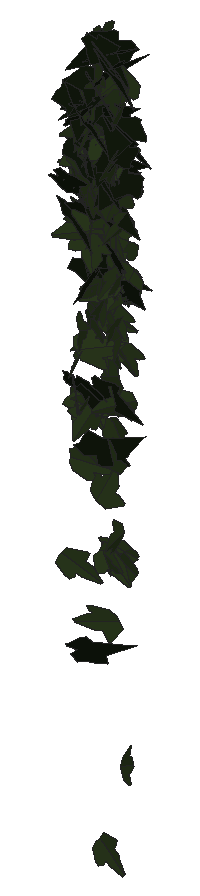
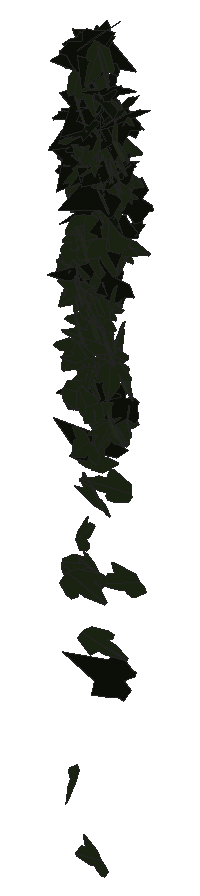
# SketchUp Ruby script. Lengths in inches.
U = 1.inch
M = Sketchup.active_model
def pt(a) = Geom::Point3d.new(a.map { |v| v * U })
def face(e, loops, mat)
  f = e.add_face(loops[0].map { |a| pt(a) })
  loops[1..].each { |l| e.add_face(l.map { |a| pt(a) }).erase! }
  f.material = f.back_material = mat if mat
  f
end
# faces: each face lists its corners as indices into pts; further lists are holes
def faces(e, pts, list, mat = nil) = list.each { |f| face(e, (f[0].is_a?(Array) ? f : [f]).map { |l| l.map { |i| pts[i] } }, mat) }
# xy, xz, yz: faces in a plane at the given z, y or x. An outline is a flat list of corners, or four numbers for a rectangle; further outlines are holes
def ring(l) = l.size == 4 ? [[l[0], l[1]], [l[2], l[1]], [l[2], l[3]], [l[0], l[3]]] : l.each_slice(2).to_a
def flat(e, list, mat, &to3) = list.each { |f| face(e, (f[0].is_a?(Array) ? f : [f]).map { |l| ring(l).map { |u, v| to3.(u, v) } }, mat) }
def xy(e, z, list, mat = nil) = flat(e, list, mat) { |x, y| [x, y, z] }
def xz(e, y, list, mat = nil) = flat(e, list, mat) { |x, z| [x, y, z] }
def yz(e, x, list, mat = nil) = flat(e, list, mat) { |y, z| [x, y, z] }
def lines(e, pts, list) = list.each { |a, b| e.add_line(pt(pts[a]), pt(pts[b])) }
# prism: a flat outline (further loops are holes) pulled along v
def prism(e, loops, v, mat = nil)
  f = face(e, loops, mat); d = Geom::Vector3d.new(v.map { |x| x * U })
  f.pushpull(f.normal.samedirection?(d) ? d.length : -d.length)
end
def box(e, o, s, mat = nil) = prism(e, [[o, [o[0] + s[0], o[1], o[2]], [o[0] + s[0], o[1] + s[1], o[2]], [o[0], o[1] + s[1], o[2]]]], [0, 0, s[2]], mat)
def at(x, y, z, deg = 0) = Geom::Transformation.translation(pt([x, y, z])) * Geom::Transformation.rotation(ORIGIN, Z_AXIS, deg.degrees)
def axes(o, x, y, z) = Geom::Transformation.new([*x, 0, *y, 0, *z, 0, *pt(o).to_a, 1])
def part(name) = M.definitions.add(name)
# library, detail: a bought-in or finely detailed component or shape, given as its bounding box
def library(name, o, s) = part(name).tap { |d| box(d.entities, o, s) }
def detail(e, o, s) = box(e.add_group.entities, o, s)
def put(e, d, t, mat = nil) = e.add_instance(d, t).tap { |i| i.material = mat if mat }
def group(e, t, mat = nil) = e.add_group.tap { |g| g.transformation = t; g.material = mat if mat }.entities
root = M.entities
M.materials.add("1026 AP 7946 SUNNY SIDE UP").color = [254, 231, 186]
M.materials.add("efeu1").color = [18, 25, 13]
M.materials.add("efeu2").color = [43, 57, 29]
c1 = part("ivyleaf_9")
p = [[1.54,2.16,1.25],[1.36,2.04,1.19],[-0.21,0.99,0.68],[-0.71,1.11,0.82],[-0.85,0.86,0.67],[-0.8,0.17,0.21],
  [-0.9,-0.01,0.1],[-0.67,-0.16,-0.02],[-0.08,-0.08,-0.05],[-0.03,-0.6,-0.4],[0.65,-0.88,-0.66],[0.83,-0.6,-0.49],
  [1.29,-0.42,-0.43],[1.8125,-0.07,-0.26],[1.21,0.44,0.15]]
faces(c1.entities,p,[[0,1,2,3,4,5,6,7,8,9,10,11,12,13,14]],"efeu1")
c2 = part("ivyleaf_10")
p = [[0,0.5,-0.03],[-0.0625,2.02,-0.43],[-0.19,2.01,-0.46],[-0.54,1.05,-0.29],[-0.52,0.625,-0.18],[-0.83,0.76,-0.28],
  [-1.16,0.64,-0.33],[-1.15,0.33,-0.24],[-0.77,-0.39,0.02],[-0.3,-0.51,0.16],[0.04,-0.48,0.23],[-0.02,2.01,-0.4375],
  [-0.06,2.01,-0.43],[0.04,-0.49,0.23],[0.67,-0.49,0.14],[1.38,0.36,-0.2],[1.375,0.51,-0.24],[0.81,0.65,-0.19],
  [0.62,0.59,-0.15],[0.6,1.09,-0.28],[0.5,1.23,-0.31]]
faces(c2.entities,p,[[0,1,2,3,4,5,6,7,8,9,10],[11,12,0,13,14,15,16,17,18,19,20]],"efeu2")
put(root,c1,axes([109.72,212.76,263.63],[0.13079,-0.20929,0.09165],[0.04808,-0.08485,-0.23249],[0.35508,0.08858,-0.00228]),"1026 AP 7946 SUNNY SIDE UP")
put(root,c2,axes([109.74,212.79,260.34],[0.07065,-0.07555,0.22326],[0.25364,-0.1473,-0.08805],[0.2576,0.16575,0.02546]),"1026 AP 7946 SUNNY SIDE UP")
put(root,c2,axes([109.94,212.7,261.06],[0.13125,-0.20202,0.03417],[0.00222,-0.03649,-0.22504],[0.32221,0.08255,-0.01237]),"1026 AP 7946 SUNNY SIDE UP")
put(root,c2,axes([109.89,212.84,264.64],[0.26049,0.1733,-0.05289],[-0.04276,-0.0463,-0.24695],[-0.28142,0.16745,-0.01144]),"1026 AP 7946 SUNNY SIDE UP")
put(root,c1,axes([109.86,212.83,265.76],[-0.08825,-0.23856,0.02828],[-0.00223,-0.02925,-0.25259],[0.37783,-0.0559,0.00512]),"1026 AP 7946 SUNNY SIDE UP")
put(root,c2,axes([110,212.6875,265.18],[0.18954,-0.20786,-0.07168],[-0.07557,0.05103,-0.24673],[0.33568,0.12886,-0.01508]),"1026 AP 7946 SUNNY SIDE UP")
put(root,c2,axes([110.16,212.74,263.43],[-0.1369,-0.00315,0.23171],[-0.24327,-0.17426,-0.06522],[0.25678,-0.16676,0.06174]),"1026 AP 7946 SUNNY SIDE UP")
put(root,c2,axes([109.96,212.96,261.23],[-0.12139,-0.20108,-0.05585],[0.03397,0.04854,-0.2216],[0.32524,-0.08012,0.0023]),"1026 AP 7946 SUNNY SIDE UP")
put(root,c1,axes([109.67,212.59,264.29],[0.36648,-0.04555,0.08565],[0.12006,-0.04172,-0.24355],[0.08895,0.244,-0.02413]),"1026 AP 7946 SUNNY SIDE UP")
put(root,c2,axes([109.97,212.83,265.22],[-0.195,-0.21529,-0.00433],[0.04409,-0.01274,-0.25407],[0.33567,-0.12339,0.03086]),"1026 AP 7946 SUNNY SIDE UP")
put(root,c2,axes([110.05,212.79,264.6],[-0.29975,-0.13813,0.05648],[-0.05119,-0.04948,-0.2419],[0.22846,-0.19231,0.0199]),"1026 AP 7946 SUNNY SIDE UP")
put(root,c2,axes([110.04,212.93,263.4375],[-0.31434,-0.10846,0.05691],[-0.0484,-0.05893,-0.23169],[0.18563,-0.19903,0.03597]),"1026 AP 7946 SUNNY SIDE UP")
put(root,c2,axes([109.83,212.97,265.43],[0.12638,-0.09056,0.21745],[0.18821,-0.17498,-0.12502],[0.30911,0.14357,-0.01278]),"1026 AP 7946 SUNNY SIDE UP")
put(root,c2,axes([109.97,212.9,264.94],[0.19883,-0.20933,-0.02797],[0.00715,0.03297,-0.25083],[0.33159,0.12481,0.02218]),"1026 AP 7946 SUNNY SIDE UP")
put(root,c2,axes([110.01,212.83,262.58],[-0.14678,0.20903,0.05276],[-0.07727,0.03234,-0.23348],[-0.329,-0.10085,0.0313]),"1026 AP 7946 SUNNY SIDE UP")
put(root,c1,axes([109.87,212.89,264.8],[0.01269,-0.2439,0.02232],[0.00005,-0.02306,-0.25153],[0.38522,0.00804,-0.0007]),"1026 AP 7946 SUNNY SIDE UP")
put(root,c2,axes([110.02,213,261.83],[0.1239,-0.20898,0.00095],[0.00598,-0.00082,-0.23007],[0.32857,0.07882,0.00383]),"1026 AP 7946 SUNNY SIDE UP")
put(root,c1,axes([109.81,212.83,265.95],[0.18215,-0.21944,-0.03716],[0.0086,0.04208,-0.25417],[0.34927,0.11341,0.02564]),"1026 AP 7946 SUNNY SIDE UP")
put(root,c2,axes([109.99,212.92,263.53],[-0.33875,0.07546,0.06254],[0.09273,-0.01392,0.23499],[0.12026,0.22328,-0.00503]),"1026 AP 7946 SUNNY SIDE UP")
put(root,c2,axes([110.02,212.76,260.19],[0.2646,0.12276,-0.07104],[-0.06702,-0.05913,-0.21379],[-0.21157,0.17226,-0.02112]),"1026 AP 7946 SUNNY SIDE UP")
put(root,c2,axes([110.19,212.78,265.2],[0.19235,-0.11093,-0.18515],[-0.20284,0.12428,-0.16935],[0.26188,0.17774,0.00482]),"1026 AP 7946 SUNNY SIDE UP")
put(root,c2,axes([110.09,212.73,263.49],[0.1737,-0.17874,-0.12958],[-0.05015,0.12512,-0.21301],[0.33906,0.11007,0.03488]),"1026 AP 7946 SUNNY SIDE UP")
put(root,c2,axes([110.06,212.86,264.89],[0.13038,-0.22595,0.05083],[0.01222,-0.05102,-0.24804],[0.36389,0.08267,-0.00988]),"1026 AP 7946 SUNNY SIDE UP")
put(root,c2,axes([110.07,212.77,260.25],[0.10919,-0.21636,0.03396],[0.00256,-0.03536,-0.23411],[0.34443,0.06886,-0.00903]),"1026 AP 7946 SUNNY SIDE UP")
put(root,c2,axes([110.01,212.75,264.88],[-0.12133,0.21466,-0.0854],[0.01343,-0.08598,-0.23462],[-0.36228,-0.07508,0.0199]),"1026 AP 7946 SUNNY SIDE UP")
put(root,c2,axes([110.06,212.56,264.42],[-0.31214,0.13505,-0.00457],[-0.01055,-0.01909,-0.24664],[-0.21225,-0.19766,0.01899]),"1026 AP 7946 SUNNY SIDE UP")
put(root,c1,axes([110.14,212.72,263.78],[0.24918,0.10255,-0.15469],[-0.21904,-0.06073,-0.19379],[-0.18493,0.21011,0.02111]),"1026 AP 7946 SUNNY SIDE UP")
put(root,c2,axes([110.14,212.8,261.67],[-0.24967,0.14445,0.06378],[-0.10517,0.01627,-0.21862],[-0.22307,-0.16935,0.03169]),"1026 AP 7946 SUNNY SIDE UP")
put(root,c2,axes([110.11,212.85,264.32],[-0.24381,-0.17738,0.06823],[0.0098,-0.09156,-0.23457],[0.29813,-0.14206,0.06351]),"1026 AP 7946 SUNNY SIDE UP")
put(root,c1,axes([109.9,212.82,265.01],[0.3859,0.01875,-0.00177],[-0.00389,0.00838,-0.25336],[-0.02937,0.24528,0.01023]),"1026 AP 7946 SUNNY SIDE UP")
put(root,c1,axes([109.83,212.9,264.9],[0.25725,-0.17887,0.03762],[0.04248,-0.02615,-0.24987],[0.28423,0.1658,0.0033]),"1026 AP 7946 SUNNY SIDE UP")
put(root,c1,axes([109.96,212.63,260.59],[0.37147,-0.01153,-0.0725],[-0.11178,-0.02184,-0.24251],[0.00751,0.24552,-0.02353]),"1026 AP 7946 SUNNY SIDE UP")
put(root,c1,axes([110.13,212.72,265.74],[0.19791,0.18578,-0.10609],[-0.08308,-0.08982,-0.23162],[-0.32432,0.13637,-0.0054]),"1026 AP 7946 SUNNY SIDE UP")
put(root,c2,axes([110.125,212.48,261.67],[0.07428,-0.10061,-0.21613],[0.01805,0.21426,-0.10222],[0.3646,0.00989,0.04909]),"1026 AP 7946 SUNNY SIDE UP")
put(root,c2,axes([109.85,212.55,257.27],[0.15202,0.03576,0.20935],[0.29884,0.07139,-0.10577],[-0.12554,0.21323,0.00172]),"1026 AP 7946 SUNNY SIDE UP")
put(root,c1,axes([110.11,212.52,265.66],[0.13967,0.21436,0.09141],[0.06154,0.07848,-0.23851],[-0.35882,0.0969,-0.00533]),"1026 AP 7946 SUNNY SIDE UP")
put(root,c2,axes([110.11,212.65,265.84],[0.31429,-0.15394,0.00427],[-0.0072,-0.01416,-0.25958],[0.24207,0.19944,-0.01327]),"1026 AP 7946 SUNNY SIDE UP")
put(root,c2,axes([110.15,212.72,260.01],[-0.11766,-0.16357,0.1602],[0.02148,-0.16772,-0.17492],[0.35523,-0.04403,0.06364]),"1026 AP 7946 SUNNY SIDE UP")
put(root,c2,axes([110.15,212.96,266.89],[0.18599,-0.21723,-0.05047],[-0.01253,0.04991,-0.25395],[0.34951,0.11739,0.01775]),"1026 AP 7946 SUNNY SIDE UP")
put(root,c2,axes([110.21,212.875,262.02],[0.22369,-0.12293,-0.14079],[-0.11804,0.11794,-0.19008],[0.26293,0.15753,0.03445]),"1026 AP 7946 SUNNY SIDE UP")
put(root,c2,axes([110.08,212.88,260.14],[0.05062,0.21389,0.0488],[0.00632,0.04606,-0.22255],[-0.34401,0.03232,0.00309]),"1026 AP 7946 SUNNY SIDE UP")
put(root,c1,axes([110.3,212.75,266.02],[-0.3004,0.11873,-0.1105],[0.07761,-0.1162,-0.22237],[-0.24008,-0.18613,0.06638]),"1026 AP 7946 SUNNY SIDE UP")
put(root,c2,axes([110.17,212.99,266.93],[-0.05677,-0.19428,-0.19837],[0.05551,0.18817,-0.20247],[0.42528,-0.0505,-0.00005]),"1026 AP 7946 SUNNY SIDE UP")
put(root,c2,axes([109.89,212.78,259.02],[-0.01548,0.0145,0.2404],[0.32924,0.10428,0.00304],[-0.16327,0.2089,-0.01667]),"1026 AP 7946 SUNNY SIDE UP")
put(root,c2,axes([110.1,212.86,264.7],[-0.28958,-0.14926,-0.07113],[0.16554,-0.02883,-0.22805],[0.19794,-0.19426,0.08667]),"1026 AP 7946 SUNNY SIDE UP")
put(root,c2,axes([110.22,212.89,264.62],[0.13468,-0.2271,-0.03328],[0.00031,0.03319,-0.24955],[0.36041,0.08483,0.01265]),"1026 AP 7946 SUNNY SIDE UP")
put(root,c2,axes([110.22,212.86,262.33],[-0.08569,-0.21964,-0.02362],[0.02689,0.01806,-0.23269],[0.346,-0.0558,0.01224]),"1026 AP 7946 SUNNY SIDE UP")
put(root,c2,axes([110.28,212.76,260.3125],[-0.25209,-0.14702,0.0398],[-0.03134,-0.03655,-0.22389],[0.23731,-0.16101,0.01271]),"1026 AP 7946 SUNNY SIDE UP")
put(root,c2,axes([110.43,212.85,256.2],[0.16178,-0.00491,-0.20985],[-0.31906,0.01802,-0.10594],[0.02876,0.22747,0.0052]),"1026 AP 7946 SUNNY SIDE UP")
put(root,c2,axes([110.25,212.89,265.07],[-0.18119,-0.21778,-0.01531],[0.02397,0.00733,-0.25358],[0.34227,-0.1158,0.00966]),"1026 AP 7946 SUNNY SIDE UP")
put(root,c1,axes([109.95,212.71,255.55],[0.2357,0.14291,-0.13636],[0.1064,0.11949,0.21125],[0.28814,-0.16102,0.03354]),"1026 AP 7946 SUNNY SIDE UP")
put(root,c2,axes([110.37,212.7,264.63],[-0.32201,0.07011,0.11018],[-0.18098,-0.0147,-0.218],[-0.08645,-0.23038,0.04597]),"1026 AP 7946 SUNNY SIDE UP")
put(root,c2,axes([110.26,212.74,266.51],[-0.24837,0.20213,-0.00499],[-0.0688,-0.04158,-0.25717],[-0.31043,-0.1525,0.06098]),"1026 AP 7946 SUNNY SIDE UP")
put(root,c2,axes([110.27,212.92,262.33],[-0.34788,0.04702,0.01628],[-0.02994,-0.01514,-0.2323],[-0.07188,-0.22127,0.01799]),"1026 AP 7946 SUNNY SIDE UP")
put(root,c2,axes([110.25,212.95,262.01],[0.05532,-0.22112,0.02292],[0.00046,-0.02375,-0.23077],[0.34964,0.03501,-0.00332]),"1026 AP 7946 SUNNY SIDE UP")
put(root,c2,axes([110.35,212.97,262.34],[0.12589,0.07172,-0.20639],[-0.22293,-0.14223,-0.11143],[-0.25032,0.16273,-0.00456]),"1026 AP 7946 SUNNY SIDE UP")
put(root,c1,axes([110.1,212.87,264.4],[0.21866,0.14211,0.1836],[0.19985,0.12382,-0.20409],[-0.29634,0.18837,-0.00216]),"1026 AP 7946 SUNNY SIDE UP")
put(root,c1,axes([110.22,212.91,266.17],[-0.18685,-0.22147,-0.01502],[0.03216,0.00411,-0.25837],[0.34738,-0.1195,0.01584]),"1026 AP 7946 SUNNY SIDE UP")
put(root,c1,axes([110.26,212.36,262.48],[0.0585,0.09433,0.24507],[0.12983,0.22253,-0.10315],[-0.38004,0.09054,0.00249]),"1026 AP 7946 SUNNY SIDE UP")
put(root,c1,axes([110.45,212.72,264.23],[-0.14774,0.22218,0.01512],[-0.03422,0.00532,-0.24779],[-0.34831,-0.09476,0.01793]),"1026 AP 7946 SUNNY SIDE UP")
put(root,c2,axes([110.32,212.82,263.27],[-0.27533,-0.15792,0.01302],[0.00199,-0.02156,-0.24242],[0.24921,-0.1743,0.01632]),"1026 AP 7946 SUNNY SIDE UP")
put(root,c1,axes([110.04,212.73,265.47],[0.19459,-0.20051,0.0869],[0.05342,-0.07937,-0.24289],[0.33855,0.12777,-0.01163]),"1026 AP 7946 SUNNY SIDE UP")
put(root,c2,axes([110.48,213.1875,257.37],[-0.18536,-0.09033,0.17569],[-0.19294,-0.11994,-0.15307],[0.23515,-0.16962,0.0129]),"1026 AP 7946 SUNNY SIDE UP")
put(root,c2,axes([110.35,212.88,262.45],[-0.20763,-0.19168,-0.0044],[0.01316,-0.0019,-0.23966],[0.30116,-0.13207,0.00744]),"1026 AP 7946 SUNNY SIDE UP")
put(root,c2,axes([110.1875,212.65,263.28],[0.36234,-0.00703,0.07593],[0.11395,-0.02864,-0.23626],[0.02418,0.24025,-0.02452]),"1026 AP 7946 SUNNY SIDE UP")
put(root,c2,axes([110.3,212.9,264.3],[0.26744,-0.17249,0.00507],[0.02904,0.00996,-0.24863],[0.26982,0.16989,0.02174]),"1026 AP 7946 SUNNY SIDE UP")
put(root,c2,axes([110.31,212.94,265.31],[-0.28185,0.15949,-0.04664],[0.02695,-0.04982,-0.24608],[-0.25969,-0.17827,0.02508]),"1026 AP 7946 SUNNY SIDE UP")
put(root,c2,axes([110.31,212.8,265.45],[0.21852,-0.1933,0.08066],[0.05455,-0.07268,-0.24529],[0.32402,0.1426,-0.0131]),"1026 AP 7946 SUNNY SIDE UP")
put(root,c1,axes([110.5,212.9375,266.96],[-0.03692,0.05146,-0.27915],[-0.02061,-0.27214,-0.05361],[-0.43365,0.00855,0.02632]),"1026 AP 7946 SUNNY SIDE UP")
put(root,c2,axes([110.42,212.91,266.25],[-0.14854,-0.22999,0.01109],[0.00153,-0.01344,-0.25615],[0.36213,-0.09428,0.00563]),"1026 AP 7946 SUNNY SIDE UP")
put(root,c1,axes([110.05,212.8,262.81],[0.10733,-0.00602,-0.2711],[0.28364,0.19901,0.04468],[0.30135,-0.18517,0.0545]),"1026 AP 7946 SUNNY SIDE UP")
put(root,c1,axes([110.41,212.73,266.76],[0.17888,0.21064,0.07292],[-0.01899,0.08397,-0.24102],[-0.3483,0.1036,0.05059]),"1026 AP 7946 SUNNY SIDE UP")
put(root,c2,axes([110.36,212.83,265.25],[-0.29233,0.15894,-0.04355],[0.03476,-0.04045,-0.25167],[-0.25664,-0.18653,0.01552]),"1026 AP 7946 SUNNY SIDE UP")
put(root,c2,axes([110.4,212.47,264.27],[-0.0645,0.21253,0.11466],[-0.06718,0.10341,-0.22144],[-0.37032,-0.05578,0.0202]),"1026 AP 7946 SUNNY SIDE UP")
put(root,c2,axes([110.14,212.62,261.27],[0.18477,-0.04865,-0.20882],[0.32559,0.05137,0.11142],[0.03389,-0.22835,0.06809]),"1026 AP 7946 SUNNY SIDE UP")
put(root,c2,axes([110.36,212.93,261.11],[0.05952,0.21953,-0.01941],[-0.00067,-0.02031,-0.22959],[-0.34663,0.03773,-0.00289]),"1026 AP 7946 SUNNY SIDE UP")
put(root,c2,axes([110.45,212.96,262.32],[0.18631,-0.19302,-0.02314],[-0.03506,0.01135,-0.23287],[0.30334,0.11986,-0.0127]),"1026 AP 7946 SUNNY SIDE UP")
put(root,c1,axes([110.22,212.84,266],[0.04119,-0.14603,0.227],[0.09862,-0.21253,-0.15345],[0.40491,0.06662,0.01428]),"1026 AP 7946 SUNNY SIDE UP")
put(root,c2,axes([110.16,213.01,261.7],[0.00579,-0.00167,0.22908],[0.33864,0.05547,-0.00292],[-0.08716,0.21538,0.00387]),"1026 AP 7946 SUNNY SIDE UP")
put(root,c2,axes([110.41,212.8125,262.49],[-0.02762,0.22622,-0.03079],[-0.02954,-0.03259,-0.23293],[-0.35785,-0.01477,0.0216]),"1026 AP 7946 SUNNY SIDE UP")
put(root,c2,axes([110.52,212.85,264.26],[-0.21444,-0.18224,0.08657],[-0.0303,-0.09047,-0.23202],[0.31478,-0.13286,0.03664]),"1026 AP 7946 SUNNY SIDE UP")
put(root,c2,axes([110.48,212.81,264.75],[-0.01645,-0.18984,0.15434],[0.01458,-0.15124,-0.19623],[0.38103,-0.00241,0.01417]),"1026 AP 7946 SUNNY SIDE UP")
put(root,c1,axes([110.26,212.76,264.66],[0.14799,-0.2213,0.02022],[0.019,-0.01755,-0.24781],[0.349,0.09479,0.00492]),"1026 AP 7946 SUNNY SIDE UP")
put(root,c2,axes([110.39,212.97,261.92],[-0.3242,0.02278,-0.08434],[0.11613,-0.05888,-0.20851],[-0.06648,-0.21393,0.04705]),"1026 AP 7946 SUNNY SIDE UP")
put(root,c2,axes([110.27,212.79,264.76],[0.27979,0.05188,-0.16866],[0.21959,0.09422,0.18734],[0.15794,-0.2229,0.03832]),"1026 AP 7946 SUNNY SIDE UP")
put(root,c2,axes([110.67,212.79,266.35],[-0.24096,0.12998,0.15117],[-0.27235,-0.00428,-0.18338],[-0.1425,-0.21162,0.09486]),"1026 AP 7946 SUNNY SIDE UP")
put(root,c1,axes([110.46,212.86,265.07],[-0.23146,-0.19562,-0.01582],[0.03684,0.00015,-0.25148],[0.3062,-0.14789,0.0183]),"1026 AP 7946 SUNNY SIDE UP")
put(root,c1,axes([110.28,212.86,264.03],[0.08771,-0.19308,-0.13953],[0.07404,0.14444,-0.19287],[0.36237,0.01722,0.07318]),"1026 AP 7946 SUNNY SIDE UP")
put(root,c2,axes([110.48,212.92,261.2],[-0.18282,0.19044,-0.02153],[-0.01994,-0.03329,-0.22824],[-0.30078,-0.11355,0.02822]),"1026 AP 7946 SUNNY SIDE UP")
put(root,c1,axes([110.31,212.93,265.63],[0.2592,-0.17718,-0.04984],[-0.04539,0.03783,-0.24905],[0.2848,0.16729,0.00567]),"1026 AP 7946 SUNNY SIDE UP")
put(root,c2,axes([110.37,212.75,258.59],[0.35633,-0.13587,-0.03688],[0.06905,0.00547,0.2708],[-0.20954,-0.22924,0.02651]),"1026 AP 7946 SUNNY SIDE UP")
put(root,c2,axes([110.7,212.7,260.9],[-0.14536,0.08612,0.19821],[-0.28728,0.07101,-0.12308],[-0.16392,-0.20083,0.03994]),"1026 AP 7946 SUNNY SIDE UP")
put(root,c2,axes([110.43,212.9,261.2],[0.3293,0.05624,-0.05837],[0.06069,0.06888,0.21658],[0.1103,-0.20582,0.05511]),"1026 AP 7946 SUNNY SIDE UP")
put(root,c2,axes([110.42,212.95,262.41],[0.3116,-0.10466,0.05097],[0.08994,0.00192,-0.22909],[0.15872,0.20439,0.02976]),"1026 AP 7946 SUNNY SIDE UP")
put(root,c2,axes([110.53,212.89,263.68],[-0.21286,-0.19459,-0.01108],[0.05853,-0.0143,-0.24101],[0.30071,-0.13496,0.03907]),"1026 AP 7946 SUNNY SIDE UP")
put(root,c2,axes([110.56,212.67,259.26],[-0.35412,0.00225,0.00456],[0.00722,0.01963,0.23125],[0.00292,0.22439,-0.01895]),"1026 AP 7946 SUNNY SIDE UP")
put(root,c2,axes([110.68,212.75,263.43],[-0.03449,0.14458,0.19442],[-0.2359,0.13765,-0.12635],[-0.28866,-0.12977,0.08003]),"1026 AP 7946 SUNNY SIDE UP")
put(root,c1,axes([110.38,212.65,267.05],[0.1497,-0.21774,-0.10033],[-0.02594,0.09727,-0.24319],[0.37337,0.09406,0.02333]),"1026 AP 7946 SUNNY SIDE UP")
put(root,c2,axes([110.36,212.87,257.41],[-0.033,0.01138,-0.23258],[0.22097,-0.17702,-0.02367],[-0.27854,-0.14178,0.00877]),"1026 AP 7946 SUNNY SIDE UP")
put(root,c2,axes([110.75,212.76,260.42],[-0.2723,0.03654,0.1431],[-0.2192,0.00827,-0.18151],[-0.05305,-0.22171,0.01547]),"1026 AP 7946 SUNNY SIDE UP")
put(root,c2,axes([110.81,212.89,257.27],[-0.14282,0.03573,-0.21374],[-0.28437,0.10288,0.10032],[0.1701,0.20199,-0.01176]),"1026 AP 7946 SUNNY SIDE UP")
put(root,c2,axes([110.6,212.875,261.82],[0.06473,-0.21913,0.03652],[0.00168,-0.03713,-0.22983],[0.34935,0.04078,-0.00566]),"1026 AP 7946 SUNNY SIDE UP")
put(root,c1,axes([110.47,212.68,265.74],[0.2524,0.17104,0.07292],[0.1037,0.03333,-0.24016],[-0.27134,0.17184,-0.02396]),"1026 AP 7946 SUNNY SIDE UP")
put(root,c2,axes([110.65,212.9375,262.47],[-0.17679,0.17079,0.10065],[-0.11847,0.06538,-0.20876],[-0.28499,-0.13313,0.02435]),"1026 AP 7946 SUNNY SIDE UP")
put(root,c2,axes([110.41,212.98,259.76],[0.24813,-0.08224,0.14287],[0.22932,-0.01142,-0.1774],[0.1096,0.21008,0.04771]),"1026 AP 7946 SUNNY SIDE UP")
put(root,c2,axes([110.49,212.76,265.13],[0.2568,0.21172,0.03202],[0.05268,0.0118,-0.27468],[-0.33205,0.16561,-0.01881]),"1026 AP 7946 SUNNY SIDE UP")
put(root,c1,axes([110.33,212.62,260.61],[0.01004,-0.01098,-0.24867],[0.30988,0.13985,-0.00037],[0.21968,-0.19677,0.01188]),"1026 AP 7946 SUNNY SIDE UP")
put(root,c2,axes([110.68,212.68,264.25],[-0.27834,-0.15079,0.04416],[-0.03216,-0.04318,-0.23899],[0.24476,-0.17715,0.01882]),"1026 AP 7946 SUNNY SIDE UP")
put(root,c2,axes([110.6,212.95,262.5625],[0.11476,-0.20867,0.05945],[0.03213,-0.05524,-0.22806],[0.33941,0.07578,0.00149]),"1026 AP 7946 SUNNY SIDE UP")
put(root,c1,axes([110.37,212.74,266.82],[0.12223,-0.18266,0.16955],[0.1178,-0.14794,-0.20519],[0.36937,0.10763,0.00933]),"1026 AP 7946 SUNNY SIDE UP")
put(root,c2,axes([110.69,212.71,261.61],[0.16358,-0.14933,-0.13628],[-0.09494,0.11763,-0.18622],[0.29806,0.11943,0.01548]),"1026 AP 7946 SUNNY SIDE UP")
put(root,c2,axes([110.43,212.88,257.37],[0.2605,0.09365,0.12891],[0.18004,0.05026,-0.19546],[-0.16631,0.20111,-0.00967]),"1026 AP 7946 SUNNY SIDE UP")
put(root,c2,axes([110.64,212.89,262.55],[0.16786,-0.20224,0.0003],[-0.00406,-0.003,-0.23558],[0.31799,0.10672,-0.00317]),"1026 AP 7946 SUNNY SIDE UP")
put(root,c1,axes([110.56,212.62,266.5],[-0.04651,0.19367,-0.17076],[-0.04992,0.16388,0.20272],[0.39885,0.0431,0.00546]),"1026 AP 7946 SUNNY SIDE UP")
put(root,c2,axes([110.7,212.93,263.22],[-0.15344,-0.18119,0.11542],[-0.01488,-0.12052,-0.20808],[0.33549,-0.08821,0.04356]),"1026 AP 7946 SUNNY SIDE UP")
put(root,c2,axes([110.47,212.95,262.5],[0.18737,0.13051,0.15006],[0.16592,0.09968,-0.18128],[-0.25789,0.15895,-0.0076]),"1026 AP 7946 SUNNY SIDE UP")
put(root,c2,axes([110.85,212.73,266.51],[-0.32405,0.05627,0.13252],[-0.2203,-0.08427,-0.19424],[0.00146,-0.22767,0.10305]),"1026 AP 7946 SUNNY SIDE UP")
put(root,c1,axes([110.55,212.77,264.81],[0.31484,0.13501,0.01373],[0.04001,-0.01541,-0.24732],[-0.20941,0.20003,-0.02661]),"1026 AP 7946 SUNNY SIDE UP")
put(root,c2,axes([110.63,212.86,263.5],[0.03049,0.23658,0.0161],[-0.02532,0.01561,-0.2438],[-0.37181,0.01834,0.01792]),"1026 AP 7946 SUNNY SIDE UP")
put(root,c2,axes([110.66,212.86,265.78],[0.14294,-0.22983,0.0384],[0.02406,-0.03543,-0.25483],[0.36566,0.09218,0.00176]),"1026 AP 7946 SUNNY SIDE UP")
put(root,c1,axes([110.7,212.87,264.62],[-0.27669,-0.17087,0.01395],[0.01159,-0.0283,-0.25149],[0.26939,-0.17428,0.02514]),"1026 AP 7946 SUNNY SIDE UP")
put(root,c1,axes([110.61,212.58,263.35],[0.30809,-0.06962,-0.12833],[-0.19663,0.01678,-0.21287],[0.10697,0.23136,-0.02169]),"1026 AP 7946 SUNNY SIDE UP")
put(root,c2,axes([110.84,212.88,262.77],[-0.30425,0.08846,0.1051],[-0.2035,-0.07309,-0.18893],[-0.05847,-0.20592,0.11064]),"1026 AP 7946 SUNNY SIDE UP")
put(root,c2,axes([110.75,212.875,253.58],[-0.04919,0.08732,0.22545],[-0.16198,0.19292,-0.09356],[-0.3324,-0.10693,0.01223]),"1026 AP 7946 SUNNY SIDE UP")
put(root,c2,axes([110.64,212.92,263.62],[0.02949,-0.05676,0.237],[0.08149,-0.22454,-0.06265],[0.36408,0.05485,-0.00517]),"1026 AP 7946 SUNNY SIDE UP")
put(root,c1,axes([110.44,212.58,259.41],[-0.06058,-0.01415,0.2524],[0.38558,-0.01397,0.0388],[0.01829,0.2477,0.01807]),"1026 AP 7946 SUNNY SIDE UP")
put(root,c1,axes([110.82,212.54,265.02],[-0.36169,0.10623,-0.05092],[-0.05807,0.03902,0.26047],[0.17527,0.23215,-0.0188]),"1026 AP 7946 SUNNY SIDE UP")
put(root,c2,axes([110.64,212.93,264.6],[-0.05741,0.23725,0.03529],[-0.00797,0.03251,-0.2471],[-0.37654,-0.03686,-0.00015]),"1026 AP 7946 SUNNY SIDE UP")
put(root,c2,axes([110.74,212.57,265.12],[0.10704,-0.23018,-0.07733],[-0.04853,0.06772,-0.24668],[0.37696,0.07408,-0.0098]),"1026 AP 7946 SUNNY SIDE UP")
put(root,c1,axes([110.77,212.72,262.7],[0.26299,0.02372,-0.20008],[-0.29616,-0.05034,-0.1736],[-0.0841,0.25142,-0.01434]),"1026 AP 7946 SUNNY SIDE UP")
put(root,c2,axes([110.73,212.75,262.74],[0.11791,0.13442,-0.1742],[-0.13182,-0.14773,-0.15943],[-0.31406,0.11248,0.00152]),"1026 AP 7946 SUNNY SIDE UP")
put(root,c2,axes([110.72,212.66,264.91],[0.02288,-0.25775,-0.05738],[0.00691,0.05455,-0.26552],[0.4141,0.01333,0.0076]),"1026 AP 7946 SUNNY SIDE UP")
put(root,c2,axes([110.72,212.93,262.46],[-0.12315,-0.11426,0.18451],[0.02563,-0.19418,-0.12097],[0.33393,-0.02723,0.07733]),"1026 AP 7946 SUNNY SIDE UP")
put(root,c2,axes([110.5625,212.86,262.81],[-0.29309,0.01549,-0.14608],[0.21012,-0.06307,-0.18831],[-0.07886,-0.22561,0.04118]),"1026 AP 7946 SUNNY SIDE UP")
put(root,c2,axes([110.65,212.91,261.34],[-0.33037,0.03031,-0.07677],[0.10978,-0.03577,-0.2175],[-0.06334,-0.2201,0.02343]),"1026 AP 7946 SUNNY SIDE UP")
put(root,c1,axes([110.52,212.84,265.4],[0.37431,-0.06034,-0.00566],[-0.01656,-0.02069,-0.25203],[0.09377,0.2372,-0.02194]),"1026 AP 7946 SUNNY SIDE UP")
put(root,c2,axes([110.72,212.76,262.6875],[0.06439,-0.22477,-0.01891],[0.03234,0.02101,-0.23395],[0.35296,0.03908,0.02489]),"1026 AP 7946 SUNNY SIDE UP")
put(root,c2,axes([110.86,212.77,260.46],[-0.05556,-0.06178,0.22605],[-0.14146,-0.20063,-0.07417],[0.32992,-0.09643,0.00626]),"1026 AP 7946 SUNNY SIDE UP")
put(root,c2,axes([110.46,212.67,252.1],[0.16021,-0.0152,0.22996],[0.33646,-0.06537,-0.10554],[0.10325,0.23659,-0.01289]),"1026 AP 7946 SUNNY SIDE UP")
put(root,c1,axes([110.71,212.88,265.62],[-0.20419,-0.21405,0.00593],[0.00865,-0.01149,-0.25776],[0.33665,-0.12954,0.01023]),"1026 AP 7946 SUNNY SIDE UP")
put(root,c1,axes([110.52,212.66,266.74],[0.21239,-0.21213,0.04991],[0.01632,-0.05209,-0.25865],[0.34218,0.13416,-0.01864]),"1026 AP 7946 SUNNY SIDE UP")
put(root,c1,axes([110.84,212.8,264.68],[-0.37705,-0.04351,-0.0355],[0.05796,-0.01205,-0.25043],[0.06493,-0.24192,0.0174]),"1026 AP 7946 SUNNY SIDE UP")
put(root,c2,axes([110.76,212.75,266.16],[-0.08036,-0.24262,0.02599],[0.02771,-0.03078,-0.25446],[0.38278,-0.0487,0.02388]),"1026 AP 7946 SUNNY SIDE UP")
put(root,c2,axes([110.68,212.79,257.9],[-0.00406,-0.00226,0.23369],[0.12942,-0.21142,-0.00244],[0.33242,0.08228,0.00381]),"1026 AP 7946 SUNNY SIDE UP")
